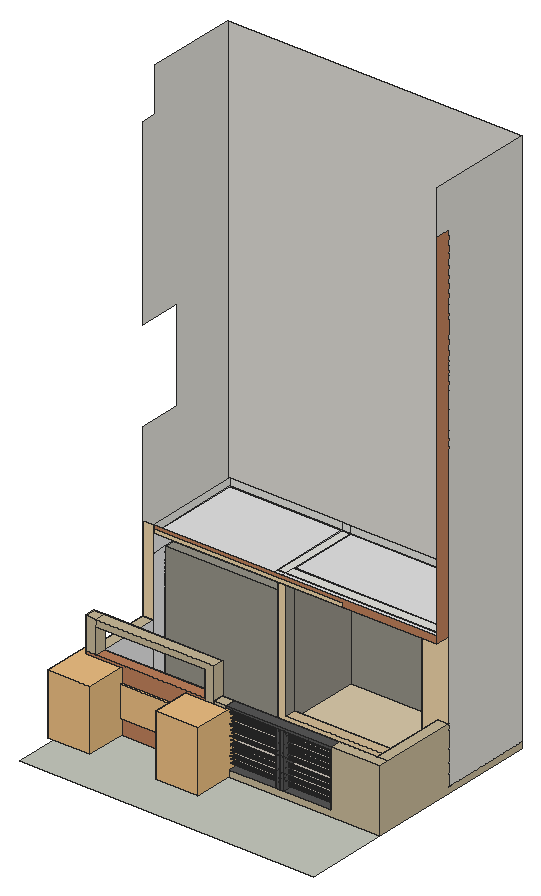
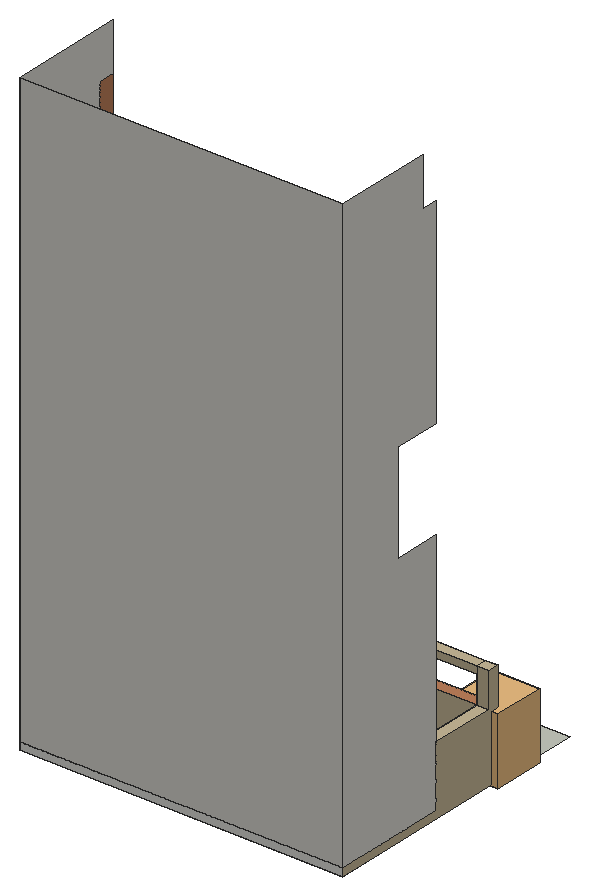
# SketchUp Ruby script. Lengths in inches.
U = 1.inch
M = Sketchup.active_model
def pt(a) = Geom::Point3d.new(a.map { |v| v * U })
def face(e, loops, mat)
  f = e.add_face(loops[0].map { |a| pt(a) })
  loops[1..].each { |l| e.add_face(l.map { |a| pt(a) }).erase! }
  f.material = f.back_material = mat if mat
  f
end
# faces: each face lists its corners as indices into pts; further lists are holes
def faces(e, pts, list, mat = nil) = list.each { |f| face(e, (f[0].is_a?(Array) ? f : [f]).map { |l| l.map { |i| pts[i] } }, mat) }
# xy, xz, yz: faces in a plane at the given z, y or x. An outline is a flat list of corners, or four numbers for a rectangle; further outlines are holes
def ring(l) = l.size == 4 ? [[l[0], l[1]], [l[2], l[1]], [l[2], l[3]], [l[0], l[3]]] : l.each_slice(2).to_a
def flat(e, list, mat, &to3) = list.each { |f| face(e, (f[0].is_a?(Array) ? f : [f]).map { |l| ring(l).map { |u, v| to3.(u, v) } }, mat) }
def xy(e, z, list, mat = nil) = flat(e, list, mat) { |x, y| [x, y, z] }
def xz(e, y, list, mat = nil) = flat(e, list, mat) { |x, z| [x, y, z] }
def yz(e, x, list, mat = nil) = flat(e, list, mat) { |y, z| [x, y, z] }
def lines(e, pts, list) = list.each { |a, b| e.add_line(pt(pts[a]), pt(pts[b])) }
# prism: a flat outline (further loops are holes) pulled along v
def prism(e, loops, v, mat = nil)
  f = face(e, loops, mat); d = Geom::Vector3d.new(v.map { |x| x * U })
  f.pushpull(f.normal.samedirection?(d) ? d.length : -d.length)
end
def box(e, o, s, mat = nil) = prism(e, [[o, [o[0] + s[0], o[1], o[2]], [o[0] + s[0], o[1] + s[1], o[2]], [o[0], o[1] + s[1], o[2]]]], [0, 0, s[2]], mat)
def at(x, y, z, deg = 0) = Geom::Transformation.translation(pt([x, y, z])) * Geom::Transformation.rotation(ORIGIN, Z_AXIS, deg.degrees)
def axes(o, x, y, z) = Geom::Transformation.new([*x, 0, *y, 0, *z, 0, *pt(o).to_a, 1])
def part(name) = M.definitions.add(name)
# library, detail: a bought-in or finely detailed component or shape, given as its bounding box
def library(name, o, s) = part(name).tap { |d| box(d.entities, o, s) }
def detail(e, o, s) = box(e.add_group.entities, o, s)
def put(e, d, t, mat = nil) = e.add_instance(d, t).tap { |i| i.material = mat if mat }
def group(e, t, mat = nil) = e.add_group.tap { |g| g.transformation = t; g.material = mat if mat }.entities
root = M.entities
M.materials.add("[Color M01]").color = [226, 226, 226]
M.materials.add("[Color M06]").color = [86, 86, 86]
M.materials.add("[Color M07]").color = [58, 58, 58]
M.materials.add("[Field Rectangle Tile]").color = [196, 189, 179]
M.materials.add("[Field Square Tile]").color = [217, 201, 169]
M.materials.add("[Formica Beige]").color = [237, 210, 167]
M.materials.add("[Formica Beige]1").color = [211, 187, 149]
M.materials.add("[Formica Graystone]").color = [149, 146, 135]
M.materials.add("[Formica Speckled Grey]").color = [94, 105, 111]
M.materials.add("[Pavers with Grass Herringbone]").color = [197, 201, 190]
M.materials.add("[Quartz Light Brown]").color = [199, 184, 152]
M.materials.add("[Terrazzo Tile Light]").color = [219, 217, 210]
M.materials.add("[Translucent Glass Blue]").color = [107, 160, 255]
M.materials["[Translucent Glass Blue]"].alpha = 0.5
M.materials.add("[Wood Veneer 02]").color = [190, 128, 91]
c1 = library("chau cay",[-24.34,-109.24,0],[56.46,62.58,79.69])
c2 = library("PANDHAN RESIDENC",[2.75,0,0],[163.32,52.5,12])
xy(root,0,[[0,107.44,386.97,341.07]])
xy(root,0,[[0,0,386.97,107.44]],"[Pavers with Grass Herringbone]")
xy(root,9,[[168.82,107.44,184.63,121.64],[250.02,107.44,255.66,121.64],[255.66,107.44,261.31,121.64],[0,201.25,0,341.07,386.97,341.07,386.97,220.875,351.34,220.875,351.34,234.35,372.59,234.35,372.59,326.6875,14.38,326.6875,14.38,201.25],[14.38,220.875,161.99,234.35],
  [161.99,220.875,173.54,326.6875],[173.54,220.875,351.34,234.35],[14.38,234.35,161.99,326.6875]])
xy(root,9,[[184.63,107.44,250.02,121.64],[261.31,107.44,323.25,121.64]],"[Color M06]")
xy(root,9,[[14.38,121.64,372.59,220.875]],"[Field Rectangle Tile]")
xy(root,9,[[173.54,234.35,372.59,326.6875]],"[Field Square Tile]")
xy(root,17.5625,[[173.54,220.875,351.34,234.35]],"[Formica Beige]1")
xy(root,79.74,[[184.63,107.44,250.02,121.64],[255.66,107.44,261.31,121.64],[261.31,107.44,323.25,121.64]])
xy(root,82.8125,[[184.63,107.44,323.25,121.64]],"[Color M06]")
xy(root,82.8125,[[168.82,107.44,184.63,121.64],[323.25,107.44,386.97,121.64],[0,121.64,14.38,201.25],[372.59,121.64,386.97,220.875]],"[Quartz Light Brown]")
xy(root,82.8125,[[14.38,107.44,157.1,121.64]],"[Wood Veneer 02]")
xy(root,116.02,[[14.38,107.44,157.1,121.64]],"[Quartz Light Brown]")
xy(root,124.4375,[[0,107.44,14.38,121.64],[14.38,107.44,168.82,121.64]],"[Quartz Light Brown]")
xy(root,161.3125,[[14.38,220.875,161.99,234.35]],"[Formica Graystone]")
xy(root,176.2,[[173.54,220.875,351.34,234.35]],"[Color M01]")
xy(root,185.25,[[161.99,220.875,173.54,326.6875],[173.54,220.875,372.59,234.35]])
xy(root,185.25,[[14.38,201.25,161.99,326.6875],[161.99,201.25,173.54,220.875],[173.54,201.25,386.97,220.875],[173.54,234.35,372.59,326.6875]],"[Color M01]")
xz(root,107.44,[[250.02,9,255.66,79.74],[255.66,9,261.31,79.74],[184.63,79.74,323.25,82.8125]],"[Color M06]")
xz(root,107.44,[[157.1,0,168.82,0,168.82,124.4375,14.38,124.4375,14.38,116.02,157.1,116.02],[168.82,0,184.63,9],[184.63,0,386.97,0,386.97,82.8125,323.25,82.8125,323.25,9,184.63,9],[168.82,9,184.63,82.8125],[0,82.8125,14.38,124.4375]],"[Quartz Light Brown]")
xz(root,107.44,[[0,0,157.1,82.8125]],"[Wood Veneer 02]")
xz(root,121.64,[[250.02,9,255.66,76.97],[255.66,9,261.31,79.74],[250.02,76.97,255.66,79.74],[184.63,79.74,323.25,82.8125]],"[Color M07]")
xz(root,121.64,[[14.38,9,14.38,82.8125,157.1,82.8125,157.1,116.02,14.38,116.02,14.38,124.4375,168.82,124.4375,168.82,9],[168.82,9,184.63,82.8125],[323.25,9,372.59,82.8125],[0,82.8125,14.38,124.4375]],"[Quartz Light Brown]")
xz(root,201.25,[[0,9,14.38,82.8125]])
xz(root,201.25,[[0,82.8125,14.38,194.875],[14.38,185.25,262.63,190.0625]],"[Formica Beige]")
xz(root,201.25,[[262.63,185.25,386.97,185.25,386.97,194.875,14.38,194.875,14.38,190.0625,262.63,190.0625]],"[Wood Veneer 02]")
xz(root,220.875,[[372.59,9,386.97,82.8125],[372.59,185.25,386.97,194.875]])
xz(root,220.875,[[161.99,9,351.34,9,351.34,17.5625,173.54,17.5625,173.54,176.2,351.34,176.2,351.34,9,372.59,9,372.59,82.8125,386.97,82.8125,386.97,185.25,161.99,185.25]],"[Formica Beige]")
xz(root,220.875,[[14.38,9,161.99,161.3125]],"[Formica Graystone]")
xz(root,234.35,[[14.38,9,161.99,161.3125],[173.54,9,351.34,17.5625],[351.34,9,372.59,176.2],[173.54,176.2,372.59,185.25]])
xz(root,326.6875,[[161.99,9,173.54,185.25],[14.38,185.25,161.99,194.875],[161.99,185.25,173.54,194.875],[173.54,185.25,372.59,194.875]])
xz(root,326.6875,[[14.38,9,161.99,185.25],[[173.54,9,372.59,185.25],[266.59,69.11,346.84,161.48]]],"[Formica Graystone]")
xz(root,326.6875,[[[266.59,69.11,346.84,161.48],[273.55,76.07,339.87,154.51]],[304.0625,76.07,309.5,154.51]],"[Formica Speckled Grey]")
xz(root,326.6875,[[273.55,76.07,304.0625,154.51],[309.5,76.07,339.87,154.51]],"[Translucent Glass Blue]")
xz(root,341.07,[[0,0,386.97,9]])
xz(root,341.07,[[0,9,386.97,722.875]],"[Terrazzo Tile Light]")
yz(root,0,[[107.44,0,107.44,124.4375,121.64,124.4375,121.64,82.8125,201.25,82.8125,201.25,9,341.07,9,341.07,0]],"[Quartz Light Brown]")
yz(root,0,[[201.25,9,201.25,305.25,257.75,305.25,257.75,425.25,201.25,425.25,201.25,665.25,221.01,665.25,221.01,722.875,341.07,722.875,341.07,9]],"[Terrazzo Tile Light]")
yz(root,14.38,[[220.875,9,234.35,161.3125],[201.25,185.25,326.6875,194.875]])
yz(root,14.38,[[121.64,9,201.25,82.8125],[201.25,9,220.875,161.3125],[234.35,9,326.6875,185.25],[201.25,161.3125,234.35,185.25]],"[Color M01]")
yz(root,14.38,[[107.44,82.8125,121.64,116.02]],"[Quartz Light Brown]")
yz(root,157.1,[[107.44,82.8125,121.64,116.02]],"[Quartz Light Brown]")
yz(root,161.99,[[220.875,9,234.35,161.3125]])
yz(root,161.99,[[234.35,9,326.6875,185.25],[220.875,161.3125,234.35,185.25]],"[Color M01]")
yz(root,168.82,[[107.44,9,121.64,82.8125]])
yz(root,168.82,[[107.44,82.8125,121.64,124.4375]],"[Quartz Light Brown]")
yz(root,173.54,[[234.35,9,326.6875,185.25],[220.875,17.5625,234.35,176.2]],"[Formica Graystone]")
yz(root,184.63,[[114.9,12.72,114.43,12.78,113.99,12.97,113.62,13.25,113.33,13.63,113.15,14.07,113.09,14.53,113.15,15,113.33,15.44,113.62,15.82,113.99,16.1,114.43,16.29,114.9,16.35,115.37,16.29,115.81,16.1,116.18,15.82,116.47,15.44,116.65,15,116.71,14.53,116.65,14.07,116.47,13.63,116.18,13.25,115.81,12.97,115.37,12.78],[114.9,20.03,114.43,20.1,113.99,20.28,113.62,20.57,113.33,20.94,113.15,21.38,113.09,21.85,113.15,22.32,113.33,22.75,113.62,23.13,113.99,23.42,114.43,23.6,114.9,23.66,115.37,23.6,115.81,23.42,116.18,23.13,116.47,22.75,116.65,22.32,116.71,21.85,116.65,21.38,116.47,20.94,116.18,20.57,115.81,20.28,115.37,20.1],[114.9,27.91,114.43,27.97,113.99,28.15,113.62,28.44,113.33,28.82,113.15,29.25,113.09,29.72,113.15,30.19,113.33,30.63,113.62,31,113.99,31.29,114.43,31.47,114.9,31.53,115.37,31.47,115.81,31.29,116.18,31,116.47,30.63,116.65,30.19,116.71,29.72,116.65,29.25,116.47,28.82,116.18,28.44,115.81,28.15,115.37,27.97],[114.9,35.16,114.43,35.22,113.99,35.4,113.62,35.69,113.33,36.07,113.15,36.5,113.09,36.97,113.15,37.44,113.33,37.88,113.62,38.25,113.99,38.54,114.43,38.72,114.9,38.78,115.37,38.72,115.81,38.54,116.18,38.25,116.47,37.88,116.65,37.44,116.71,36.97,116.65,36.5,116.47,36.07,116.18,35.69,115.81,35.4,115.37,35.22],[114.9,43.85,114.43,43.91,113.99,44.09,113.62,44.38,113.33,44.75,113.15,45.19,113.09,45.66,113.15,46.13,113.33,46.57,113.62,46.94,113.99,47.23,114.43,47.41,114.9,47.47,115.37,47.41,115.81,47.23,116.18,46.94,116.47,46.57,116.65,46.13,116.71,45.66,116.65,45.19,116.47,44.75,116.18,44.38,115.81,44.09,115.37,43.91],
  [114.9,51.66,114.43,51.72,113.99,51.9,113.62,52.19,113.33,52.57,113.15,53,113.09,53.47,113.15,53.94,113.33,54.38,113.62,54.75,113.99,55.04,114.43,55.22,114.9,55.28,115.37,55.22,115.81,55.04,116.18,54.75,116.47,54.38,116.65,53.94,116.71,53.47,116.65,53,116.47,52.57,116.18,52.19,115.81,51.9,115.37,51.72],[114.9,58.41,114.43,58.47,113.99,58.65,113.62,58.94,113.33,59.32,113.15,59.75,113.09,60.22,113.15,60.69,113.33,61.13,113.62,61.5,113.99,61.79,114.43,61.97,114.9,62.03,115.37,61.97,115.81,61.79,116.18,61.5,116.47,61.13,116.65,60.69,116.71,60.22,116.65,59.75,116.47,59.32,116.18,58.94,115.81,58.65,115.37,58.47],[114.9,65.85,114.43,65.91,113.99,66.09,113.62,66.38,113.33,66.75,113.15,67.19,113.09,67.66,113.15,68.13,113.33,68.57,113.62,68.94,113.99,69.23,114.43,69.41,114.9,69.47,115.37,69.41,115.81,69.23,116.18,68.94,116.47,68.57,116.65,68.13,116.71,67.66,116.65,67.19,116.47,66.75,116.18,66.38,115.81,66.09,115.37,65.91],[114.9,72.53,114.43,72.6,113.99,72.78,113.62,73.07,113.33,73.44,113.15,73.88,113.09,74.35,113.15,74.82,113.33,75.25,113.62,75.63,113.99,75.92,114.43,76.1,114.9,76.16,115.37,76.1,115.81,75.92,116.18,75.63,116.47,75.25,116.65,74.82,116.71,74.35,116.65,73.88,116.47,73.44,116.18,73.07,115.81,72.78,115.37,72.6],[107.44,79.74,121.64,82.8125]])
yz(root,184.63,[[[107.44,9,121.64,79.74],[114.9,12.72,114.43,12.78,113.99,12.97,113.62,13.25,113.33,13.63,113.15,14.07,113.09,14.53,113.15,15,113.33,15.44,113.62,15.82,113.99,16.1,114.43,16.29,114.9,16.35,115.37,16.29,115.81,16.1,116.18,15.82,116.47,15.44,116.65,15,116.71,14.53,116.65,14.07,116.47,13.63,116.18,13.25,115.81,12.97,115.37,12.78],[114.9,65.85,114.43,65.91,113.99,66.09,113.62,66.38,113.33,66.75,113.15,67.19,113.09,67.66,113.15,68.13,113.33,68.57,113.62,68.94,113.99,69.23,114.43,69.41,114.9,69.47,115.37,69.41,115.81,69.23,116.18,68.94,116.47,68.57,116.65,68.13,116.71,67.66,116.65,67.19,116.47,66.75,116.18,66.38,115.81,66.09,115.37,65.91],[114.9,20.03,114.43,20.1,113.99,20.28,113.62,20.57,113.33,20.94,113.15,21.38,113.09,21.85,113.15,22.32,113.33,22.75,113.62,23.13,113.99,23.42,114.43,23.6,114.9,23.66,115.37,23.6,115.81,23.42,116.18,23.13,116.47,22.75,116.65,22.32,116.71,21.85,116.65,21.38,116.47,20.94,116.18,20.57,115.81,20.28,115.37,20.1],[114.9,58.41,114.43,58.47,113.99,58.65,113.62,58.94,113.33,59.32,113.15,59.75,113.09,60.22,113.15,60.69,113.33,61.13,113.62,61.5,113.99,61.79,114.43,61.97,114.9,62.03,115.37,61.97,115.81,61.79,116.18,61.5,116.47,61.13,116.65,60.69,116.71,60.22,116.65,59.75,116.47,59.32,116.18,58.94,115.81,58.65,115.37,58.47],[114.9,27.91,114.43,27.97,113.99,28.15,113.62,28.44,113.33,28.82,113.15,29.25,113.09,29.72,113.15,30.19,113.33,30.63,113.62,31,113.99,31.29,114.43,31.47,114.9,31.53,115.37,31.47,115.81,31.29,116.18,31,116.47,30.63,116.65,30.19,116.71,29.72,116.65,29.25,116.47,28.82,116.18,28.44,115.81,28.15,115.37,27.97],[114.9,51.66,114.43,51.72,113.99,51.9,113.62,52.19,113.33,52.57,113.15,53,113.09,53.47,113.15,53.94,113.33,54.38,113.62,54.75,113.99,55.04,114.43,55.22,114.9,55.28,115.37,55.22,115.81,55.04,116.18,54.75,116.47,54.38,116.65,53.94,116.71,53.47,116.65,53,116.47,52.57,116.18,52.19,115.81,51.9,115.37,51.72],[114.9,35.16,114.43,35.22,113.99,35.4,113.62,35.69,113.33,36.07,113.15,36.5,113.09,36.97,113.15,37.44,113.33,37.88,113.62,38.25,113.99,38.54,114.43,38.72,114.9,38.78,115.37,38.72,115.81,38.54,116.18,38.25,116.47,37.88,116.65,37.44,116.71,36.97,116.65,36.5,116.47,36.07,116.18,35.69,115.81,35.4,115.37,35.22],[114.9,43.85,114.43,43.91,113.99,44.09,113.62,44.38,113.33,44.75,113.15,45.19,113.09,45.66,113.15,46.13,113.33,46.57,113.62,46.94,113.99,47.23,114.43,47.41,114.9,47.47,115.37,47.41,115.81,47.23,116.18,46.94,116.47,46.57,116.65,46.13,116.71,45.66,116.65,45.19,116.47,44.75,116.18,44.38,115.81,44.09,115.37,43.91],[114.9,72.53,114.43,72.6,113.99,72.78,113.62,73.07,113.33,73.44,113.15,73.88,113.09,74.35,113.15,74.82,113.33,75.25,113.62,75.63,113.99,75.92,114.43,76.1,114.9,76.16,115.37,76.1,115.81,75.92,116.18,75.63,116.47,75.25,116.65,74.82,116.71,74.35,116.65,73.88,116.47,73.44,116.18,73.07,115.81,72.78,115.37,72.6]]],"[Color M06]")
yz(root,250.02,[[107.44,9,121.64,76.97],[107.44,76.97,121.64,79.74]],"[Color M06]")
yz(root,255.66,[[107.44,9,121.64,76.97],[107.44,76.97,121.64,79.74]])
yz(root,261.31,[[107.44,9,121.64,79.74]],"[Color M06]")
yz(root,323.25,[[[107.44,9,121.64,79.74],[114.9,72.53,115.37,72.6,115.81,72.78,116.18,73.07,116.47,73.44,116.65,73.88,116.71,74.35,116.65,74.82,116.47,75.25,116.18,75.63,115.81,75.92,115.37,76.1,114.9,76.16,114.43,76.1,113.99,75.92,113.62,75.63,113.33,75.25,113.15,74.82,113.09,74.35,113.15,73.88,113.33,73.44,113.62,73.07,113.99,72.78,114.43,72.6],[114.9,65.85,115.37,65.91,115.81,66.09,116.18,66.38,116.47,66.75,116.65,67.19,116.71,67.66,116.65,68.13,116.47,68.57,116.18,68.94,115.81,69.23,115.37,69.41,114.9,69.47,114.43,69.41,113.99,69.23,113.62,68.94,113.33,68.57,113.15,68.13,113.09,67.66,113.15,67.19,113.33,66.75,113.62,66.38,113.99,66.09,114.43,65.91],[114.9,58.41,115.37,58.47,115.81,58.65,116.18,58.94,116.47,59.32,116.65,59.75,116.71,60.22,116.65,60.69,116.47,61.13,116.18,61.5,115.81,61.79,115.37,61.97,114.9,62.03,114.43,61.97,113.99,61.79,113.62,61.5,113.33,61.13,113.15,60.69,113.09,60.22,113.15,59.75,113.33,59.32,113.62,58.94,113.99,58.65,114.43,58.47],[114.9,51.66,115.37,51.72,115.81,51.9,116.18,52.19,116.47,52.57,116.65,53,116.71,53.47,116.65,53.94,116.47,54.38,116.18,54.75,115.81,55.04,115.37,55.22,114.9,55.28,114.43,55.22,113.99,55.04,113.62,54.75,113.33,54.38,113.15,53.94,113.09,53.47,113.15,53,113.33,52.57,113.62,52.19,113.99,51.9,114.43,51.72],[114.9,43.85,115.37,43.91,115.81,44.09,116.18,44.38,116.47,44.75,116.65,45.19,116.71,45.66,116.65,46.13,116.47,46.57,116.18,46.94,115.81,47.23,115.37,47.41,114.9,47.47,114.43,47.41,113.99,47.23,113.62,46.94,113.33,46.57,113.15,46.13,113.09,45.66,113.15,45.19,113.33,44.75,113.62,44.38,113.99,44.09,114.43,43.91],[114.9,35.16,115.37,35.22,115.81,35.4,116.18,35.69,116.47,36.07,116.65,36.5,116.71,36.97,116.65,37.44,116.47,37.88,116.18,38.25,115.81,38.54,115.37,38.72,114.9,38.78,114.43,38.72,113.99,38.54,113.62,38.25,113.33,37.88,113.15,37.44,113.09,36.97,113.15,36.5,113.33,36.07,113.62,35.69,113.99,35.4,114.43,35.22],[114.9,27.91,115.37,27.97,115.81,28.15,116.18,28.44,116.47,28.82,116.65,29.25,116.71,29.72,116.65,30.19,116.47,30.63,116.18,31,115.81,31.29,115.37,31.47,114.9,31.53,114.43,31.47,113.99,31.29,113.62,31,113.33,30.63,113.15,30.19,113.09,29.72,113.15,29.25,113.33,28.82,113.62,28.44,113.99,28.15,114.43,27.97],[114.9,20.03,115.37,20.1,115.81,20.28,116.18,20.57,116.47,20.94,116.65,21.38,116.71,21.85,116.65,22.32,116.47,22.75,116.18,23.13,115.81,23.42,115.37,23.6,114.9,23.66,114.43,23.6,113.99,23.42,113.62,23.13,113.33,22.75,113.15,22.32,113.09,21.85,113.15,21.38,113.33,20.94,113.62,20.57,113.99,20.28,114.43,20.1],[114.9,12.72,115.37,12.78,115.81,12.97,116.18,13.25,116.47,13.63,116.65,14.07,116.71,14.53,116.65,15,116.47,15.44,116.18,15.82,115.81,16.1,115.37,16.29,114.9,16.35,114.43,16.29,113.99,16.1,113.62,15.82,113.33,15.44,113.15,15,113.09,14.53,113.15,14.07,113.33,13.63,113.62,13.25,113.99,12.97,114.43,12.78]]],"[Color M06]")
yz(root,351.34,[[220.875,9,234.35,17.5625]])
yz(root,351.34,[[220.875,17.5625,234.35,176.2]],"[Formica Graystone]")
yz(root,372.59,[[220.875,185.25,326.6875,194.875]])
yz(root,372.59,[[121.64,9,220.875,82.8125]],"[Color M01]")
yz(root,372.59,[[234.35,9,326.6875,185.25]],"[Formica Graystone]")
yz(root,386.97,[[107.44,0,341.07,0,341.07,9,220.875,9,220.875,82.8125,107.44,82.8125]],"[Quartz Light Brown]")
yz(root,386.97,[[220.875,9,341.07,9,341.07,722.875,201.25,722.875,201.25,665.25,220.875,665.25]],"[Terrazzo Tile Light]")
yz(root,386.97,[[201.25,185.25,220.875,665.25]],"[Wood Veneer 02]")
p = [[184.63,114.43,12.78],[184.63,114.9,12.72],[323.25,114.9,12.72],[323.25,114.43,12.78],[184.63,115.37,12.78],[323.25,115.37,12.78],
  [184.63,113.99,12.97],[323.25,113.99,12.97],[184.63,115.81,12.97],[323.25,115.81,12.97],[184.63,113.62,13.25],[323.25,113.62,13.25],
  [184.63,116.18,13.25],[323.25,116.18,13.25],[184.63,113.33,13.63],[323.25,113.33,13.63],[184.63,116.47,13.63],[323.25,116.47,13.63],
  [184.63,113.15,14.07],[323.25,113.15,14.07],[184.63,116.65,14.07],[323.25,116.65,14.07],[184.63,113.09,14.53],[323.25,113.09,14.53],
  [184.63,116.71,14.53],[323.25,116.71,14.53],[184.63,113.15,15],[323.25,113.15,15],[184.63,116.65,15],[323.25,116.65,15],
  [184.63,113.33,15.44],[323.25,113.33,15.44],[184.63,116.47,15.44],[323.25,116.47,15.44],[184.63,113.62,15.82],[323.25,113.62,15.82],
  [184.63,116.18,15.82],[323.25,116.18,15.82],[184.63,113.99,16.1],[323.25,113.99,16.1],[184.63,115.81,16.1],[323.25,115.81,16.1],
  [184.63,114.43,16.29],[323.25,114.43,16.29],[184.63,115.37,16.29],[323.25,115.37,16.29],[184.63,114.9,16.35],[323.25,114.9,16.35],
  [184.63,114.43,20.1],[184.63,114.9,20.03],[323.25,114.9,20.03],[323.25,114.43,20.1],[184.63,115.37,20.1],[323.25,115.37,20.1],
  [184.63,113.99,20.28],[323.25,113.99,20.28],[184.63,115.81,20.28],[323.25,115.81,20.28],[184.63,113.62,20.57],[323.25,113.62,20.57],
  [184.63,116.18,20.57],[323.25,116.18,20.57],[184.63,113.33,20.94],[323.25,113.33,20.94],[184.63,116.47,20.94],[323.25,116.47,20.94],
  [184.63,113.15,21.38],[323.25,113.15,21.38],[184.63,116.65,21.38],[323.25,116.65,21.38],[184.63,113.09,21.85],[323.25,113.09,21.85],
  [184.63,116.71,21.85],[323.25,116.71,21.85],[184.63,113.15,22.32],[323.25,113.15,22.32],[184.63,116.65,22.32],[323.25,116.65,22.32],
  [184.63,113.33,22.75],[323.25,113.33,22.75],[184.63,116.47,22.75],[323.25,116.47,22.75],[184.63,113.62,23.13],[323.25,113.62,23.13],
  [184.63,116.18,23.13],[323.25,116.18,23.13],[184.63,113.99,23.42],[323.25,113.99,23.42],[184.63,115.81,23.42],[323.25,115.81,23.42],
  [184.63,114.43,23.6],[323.25,114.43,23.6],[184.63,115.37,23.6],[323.25,115.37,23.6],[184.63,114.9,23.66],[323.25,114.9,23.66],
  [184.63,114.43,27.97],[184.63,114.9,27.91],[323.25,114.9,27.91],[323.25,114.43,27.97],[184.63,115.37,27.97],[323.25,115.37,27.97],
  [184.63,113.99,28.15],[323.25,113.99,28.15],[184.63,115.81,28.15],[323.25,115.81,28.15],[184.63,113.62,28.44],[323.25,113.62,28.44],
  [184.63,116.18,28.44],[323.25,116.18,28.44],[184.63,113.33,28.82],[323.25,113.33,28.82],[184.63,116.47,28.82],[323.25,116.47,28.82],
  [184.63,113.15,29.25],[323.25,113.15,29.25],[184.63,116.65,29.25],[323.25,116.65,29.25],[184.63,113.09,29.72],[323.25,113.09,29.72],
  [184.63,116.71,29.72],[323.25,116.71,29.72],[184.63,113.15,30.19],[323.25,113.15,30.19],[184.63,116.65,30.19],[323.25,116.65,30.19],
  [184.63,113.33,30.63],[323.25,113.33,30.63],[184.63,116.47,30.63],[323.25,116.47,30.63],[184.63,113.62,31],[323.25,113.62,31],
  [184.63,116.18,31],[323.25,116.18,31],[184.63,113.99,31.29],[323.25,113.99,31.29],[184.63,115.81,31.29],[323.25,115.81,31.29],
  [184.63,114.43,31.47],[323.25,114.43,31.47],[184.63,115.37,31.47],[323.25,115.37,31.47],[184.63,114.9,31.53],[323.25,114.9,31.53],
  [184.63,113.99,35.4],[184.63,114.43,35.22],[323.25,114.43,35.22],[323.25,113.99,35.4],[184.63,114.9,35.16],[323.25,114.9,35.16],
  [184.63,115.37,35.22],[323.25,115.37,35.22],[184.63,115.81,35.4],[323.25,115.81,35.4],[184.63,113.62,35.69],[323.25,113.62,35.69],
  [184.63,116.18,35.69],[323.25,116.18,35.69],[184.63,113.33,36.07],[323.25,113.33,36.07],[184.63,116.47,36.07],[323.25,116.47,36.07],
  [184.63,113.15,36.5],[323.25,113.15,36.5],[184.63,116.65,36.5],[323.25,116.65,36.5],[184.63,113.09,36.97],[323.25,113.09,36.97],
  [184.63,116.71,36.97],[323.25,116.71,36.97],[184.63,113.15,37.44],[323.25,113.15,37.44],[184.63,116.65,37.44],[323.25,116.65,37.44],
  [184.63,113.33,37.88],[323.25,113.33,37.88],[184.63,116.47,37.88],[323.25,116.47,37.88],[184.63,113.62,38.25],[323.25,113.62,38.25],
  [184.63,116.18,38.25],[323.25,116.18,38.25],[184.63,113.99,38.54],[323.25,113.99,38.54],[184.63,115.81,38.54],[323.25,115.81,38.54],
  [184.63,114.43,38.72],[323.25,114.43,38.72],[184.63,115.37,38.72],[323.25,115.37,38.72],[184.63,114.9,38.78],[323.25,114.9,38.78],
  [184.63,114.43,43.91],[184.63,114.9,43.85],[323.25,114.9,43.85],[323.25,114.43,43.91],[184.63,115.37,43.91],[323.25,115.37,43.91],
  [184.63,113.99,44.09],[323.25,113.99,44.09],[184.63,115.81,44.09],[323.25,115.81,44.09],[184.63,113.62,44.38],[323.25,113.62,44.38],
  [184.63,116.18,44.38],[323.25,116.18,44.38],[184.63,113.33,44.75],[323.25,113.33,44.75],[184.63,116.47,44.75],[323.25,116.47,44.75],
  [184.63,113.15,45.19],[323.25,113.15,45.19],[184.63,116.65,45.19],[323.25,116.65,45.19],[184.63,113.09,45.66],[323.25,113.09,45.66],
  [184.63,116.71,45.66],[323.25,116.71,45.66],[184.63,113.15,46.13],[323.25,113.15,46.13],[184.63,116.65,46.13],[323.25,116.65,46.13],
  [184.63,113.33,46.57],[323.25,113.33,46.57],[184.63,116.47,46.57],[323.25,116.47,46.57],[184.63,113.62,46.94],[323.25,113.62,46.94],
  [184.63,116.18,46.94],[323.25,116.18,46.94],[184.63,113.99,47.23],[323.25,113.99,47.23],[184.63,115.81,47.23],[323.25,115.81,47.23],
  [184.63,114.43,47.41],[323.25,114.43,47.41],[184.63,115.37,47.41],[323.25,115.37,47.41],[184.63,114.9,47.47],[323.25,114.9,47.47],
  [184.63,113.99,51.9],[184.63,114.43,51.72],[323.25,114.43,51.72],[323.25,113.99,51.9],[184.63,114.9,51.66],[323.25,114.9,51.66],
  [184.63,115.37,51.72],[323.25,115.37,51.72],[184.63,115.81,51.9],[323.25,115.81,51.9],[184.63,113.62,52.19],[323.25,113.62,52.19],
  [184.63,116.18,52.19],[323.25,116.18,52.19],[184.63,113.33,52.57],[323.25,113.33,52.57],[184.63,116.47,52.57],[323.25,116.47,52.57],
  [184.63,113.15,53],[323.25,113.15,53],[184.63,116.65,53],[323.25,116.65,53],[184.63,113.09,53.47],[323.25,113.09,53.47],
  [184.63,116.71,53.47],[323.25,116.71,53.47],[184.63,113.15,53.94],[323.25,113.15,53.94],[184.63,116.65,53.94],[323.25,116.65,53.94],
  [184.63,113.33,54.38],[323.25,113.33,54.38],[184.63,116.47,54.38],[323.25,116.47,54.38],[184.63,113.62,54.75],[323.25,113.62,54.75],
  [184.63,116.18,54.75],[323.25,116.18,54.75],[184.63,113.99,55.04],[323.25,113.99,55.04],[184.63,115.81,55.04],[323.25,115.81,55.04],
  [184.63,114.43,55.22],[323.25,114.43,55.22],[184.63,115.37,55.22],[323.25,115.37,55.22],[184.63,114.9,55.28],[323.25,114.9,55.28],
  [184.63,114.43,58.47],[184.63,114.9,58.41],[323.25,114.9,58.41],[323.25,114.43,58.47],[184.63,115.37,58.47],[323.25,115.37,58.47],
  [184.63,113.99,58.65],[323.25,113.99,58.65],[184.63,115.81,58.65],[323.25,115.81,58.65],[184.63,113.62,58.94],[323.25,113.62,58.94],
  [184.63,116.18,58.94],[323.25,116.18,58.94],[184.63,113.33,59.32],[323.25,113.33,59.32],[184.63,116.47,59.32],[323.25,116.47,59.32],
  [184.63,113.15,59.75],[323.25,113.15,59.75],[184.63,116.65,59.75],[323.25,116.65,59.75],[184.63,113.09,60.22],[323.25,113.09,60.22],
  [184.63,116.71,60.22],[323.25,116.71,60.22],[184.63,113.15,60.69],[323.25,113.15,60.69],[184.63,116.65,60.69],[323.25,116.65,60.69],
  [184.63,113.33,61.13],[323.25,113.33,61.13],[184.63,116.47,61.13],[323.25,116.47,61.13],[184.63,113.62,61.5],[323.25,113.62,61.5],
  [184.63,116.18,61.5],[323.25,116.18,61.5],[184.63,113.99,61.79],[323.25,113.99,61.79],[184.63,115.81,61.79],[323.25,115.81,61.79],
  [184.63,114.43,61.97],[323.25,114.43,61.97],[184.63,115.37,61.97],[323.25,115.37,61.97],[184.63,114.9,62.03],[323.25,114.9,62.03],
  [184.63,114.43,65.91],[184.63,114.9,65.85],[323.25,114.9,65.85],[323.25,114.43,65.91],[184.63,115.37,65.91],[323.25,115.37,65.91],
  [184.63,113.99,66.09],[323.25,113.99,66.09],[184.63,115.81,66.09],[323.25,115.81,66.09],[184.63,113.62,66.38],[323.25,113.62,66.38],
  [184.63,116.18,66.38],[323.25,116.18,66.38],[184.63,113.33,66.75],[323.25,113.33,66.75],[184.63,116.47,66.75],[323.25,116.47,66.75],
  [184.63,113.15,67.19],[323.25,113.15,67.19],[184.63,116.65,67.19],[323.25,116.65,67.19],[184.63,113.09,67.66],[323.25,113.09,67.66],
  [184.63,116.71,67.66],[323.25,116.71,67.66],[184.63,113.15,68.13],[323.25,113.15,68.13],[184.63,116.65,68.13],[323.25,116.65,68.13],
  [184.63,113.33,68.57],[323.25,113.33,68.57],[184.63,116.47,68.57],[323.25,116.47,68.57],[184.63,113.62,68.94],[323.25,113.62,68.94],
  [184.63,116.18,68.94],[323.25,116.18,68.94],[184.63,113.99,69.23],[323.25,113.99,69.23],[184.63,115.81,69.23],[323.25,115.81,69.23],
  [184.63,114.43,69.41],[323.25,114.43,69.41],[184.63,115.37,69.41],[323.25,115.37,69.41],[184.63,114.9,69.47],[323.25,114.9,69.47],
  [184.63,114.43,72.6],[184.63,114.9,72.53],[323.25,114.9,72.53],[323.25,114.43,72.6],[184.63,115.37,72.6],[323.25,115.37,72.6],
  [184.63,113.99,72.78],[323.25,113.99,72.78],[184.63,115.81,72.78],[323.25,115.81,72.78],[184.63,113.62,73.07],[323.25,113.62,73.07],
  [184.63,116.18,73.07],[323.25,116.18,73.07],[184.63,113.33,73.44],[323.25,113.33,73.44],[184.63,116.47,73.44],[323.25,116.47,73.44],
  [184.63,113.15,73.88],[323.25,113.15,73.88],[184.63,116.65,73.88],[323.25,116.65,73.88],[184.63,113.09,74.35],[323.25,113.09,74.35],
  [184.63,116.71,74.35],[323.25,116.71,74.35],[184.63,113.15,74.82],[323.25,113.15,74.82],[184.63,116.65,74.82],[323.25,116.65,74.82],
  [184.63,113.33,75.25],[323.25,113.33,75.25],[184.63,116.47,75.25],[323.25,116.47,75.25],[184.63,113.62,75.63],[323.25,113.62,75.63],
  [184.63,116.18,75.63],[323.25,116.18,75.63],[184.63,113.99,75.92],[323.25,113.99,75.92],[184.63,115.81,75.92],[323.25,115.81,75.92],
  [184.63,114.43,76.1],[323.25,114.43,76.1],[184.63,115.37,76.1],[323.25,115.37,76.1],[184.63,114.9,76.16],[323.25,114.9,76.16]]
faces(root,p,[[0,1,2,3],[1,4,5,2],[6,0,3,7],[4,8,9,5],[10,6,7,11],[8,12,13,9],[14,10,11,15],[12,16,17,13],
  [18,14,15,19],[16,20,21,17],[22,18,19,23],[20,24,25,21],[26,22,23,27],[24,28,29,25],[30,26,27,31],[28,32,33,29],
  [34,30,31,35],[32,36,37,33],[38,34,35,39],[36,40,41,37],[42,38,39,43],[40,44,45,41],[46,42,43,47],[44,46,47,45],
  [48,49,50,51],[49,52,53,50],[54,48,51,55],[52,56,57,53],[58,54,55,59],[56,60,61,57],[62,58,59,63],[60,64,65,61],
  [66,62,63,67],[64,68,69,65],[70,66,67,71],[68,72,73,69],[74,70,71,75],[72,76,77,73],[78,74,75,79],[76,80,81,77],
  [82,78,79,83],[80,84,85,81],[86,82,83,87],[84,88,89,85],[90,86,87,91],[88,92,93,89],[94,90,91,95],[92,94,95,93],
  [96,97,98,99],[97,100,101,98],[102,96,99,103],[100,104,105,101],[106,102,103,107],[104,108,109,105],[110,106,107,111],[108,112,113,109],
  [114,110,111,115],[112,116,117,113],[118,114,115,119],[116,120,121,117],[122,118,119,123],[120,124,125,121],[126,122,123,127],[124,128,129,125],
  [130,126,127,131],[128,132,133,129],[134,130,131,135],[132,136,137,133],[138,134,135,139],[136,140,141,137],[142,138,139,143],[140,142,143,141],
  [144,145,146,147],[145,148,149,146],[148,150,151,149],[150,152,153,151],[154,144,147,155],[152,156,157,153],[158,154,155,159],[156,160,161,157],
  [162,158,159,163],[160,164,165,161],[166,162,163,167],[164,168,169,165],[170,166,167,171],[168,172,173,169],[174,170,171,175],[172,176,177,173],
  [178,174,175,179],[176,180,181,177],[182,178,179,183],[180,184,185,181],[186,182,183,187],[184,188,189,185],[190,186,187,191],[188,190,191,189],
  [192,193,194,195],[193,196,197,194],[198,192,195,199],[196,200,201,197],[202,198,199,203],[200,204,205,201],[206,202,203,207],[204,208,209,205],
  [210,206,207,211],[208,212,213,209],[214,210,211,215],[212,216,217,213],[218,214,215,219],[216,220,221,217],[222,218,219,223],[220,224,225,221],
  [226,222,223,227],[224,228,229,225],[230,226,227,231],[228,232,233,229],[234,230,231,235],[232,236,237,233],[238,234,235,239],[236,238,239,237],
  [240,241,242,243],[241,244,245,242],[244,246,247,245],[246,248,249,247],[250,240,243,251],[248,252,253,249],[254,250,251,255],[252,256,257,253],
  [258,254,255,259],[256,260,261,257],[262,258,259,263],[260,264,265,261],[266,262,263,267],[264,268,269,265],[270,266,267,271],[268,272,273,269],
  [274,270,271,275],[272,276,277,273],[278,274,275,279],[276,280,281,277],[282,278,279,283],[280,284,285,281],[286,282,283,287],[284,286,287,285],
  [288,289,290,291],[289,292,293,290],[294,288,291,295],[292,296,297,293],[298,294,295,299],[296,300,301,297],[302,298,299,303],[300,304,305,301],
  [306,302,303,307],[304,308,309,305],[310,306,307,311],[308,312,313,309],[314,310,311,315],[312,316,317,313],[318,314,315,319],[316,320,321,317],
  [322,318,319,323],[320,324,325,321],[326,322,323,327],[324,328,329,325],[330,326,327,331],[328,332,333,329],[334,330,331,335],[332,334,335,333],
  [336,337,338,339],[337,340,341,338],[342,336,339,343],[340,344,345,341],[346,342,343,347],[344,348,349,345],[350,346,347,351],[348,352,353,349],
  [354,350,351,355],[352,356,357,353],[358,354,355,359],[356,360,361,357],[362,358,359,363],[360,364,365,361],[366,362,363,367],[364,368,369,365],
  [370,366,367,371],[368,372,373,369],[374,370,371,375],[372,376,377,373],[378,374,375,379],[376,380,381,377],[382,378,379,383],[380,382,383,381],
  [384,385,386,387],[385,388,389,386],[390,384,387,391],[388,392,393,389],[394,390,391,395],[392,396,397,393],[398,394,395,399],[396,400,401,397],
  [402,398,399,403],[400,404,405,401],[406,402,403,407],[404,408,409,405],[410,406,407,411],[408,412,413,409],[414,410,411,415],[412,416,417,413],
  [418,414,415,419],[416,420,421,417],[422,418,419,423],[420,424,425,421],[426,422,423,427],[424,428,429,425],[430,426,427,431],[428,430,431,429]],"[Color M06]")
put(root,c1,at(15.46,165.35,0))
put(root,c1,at(156.09,167.16,0))
put(root,c2,axes([28.96,107.44,21.54],[0.65022,0,0],[0,0,0.77],[0,-0.27404,0]))
